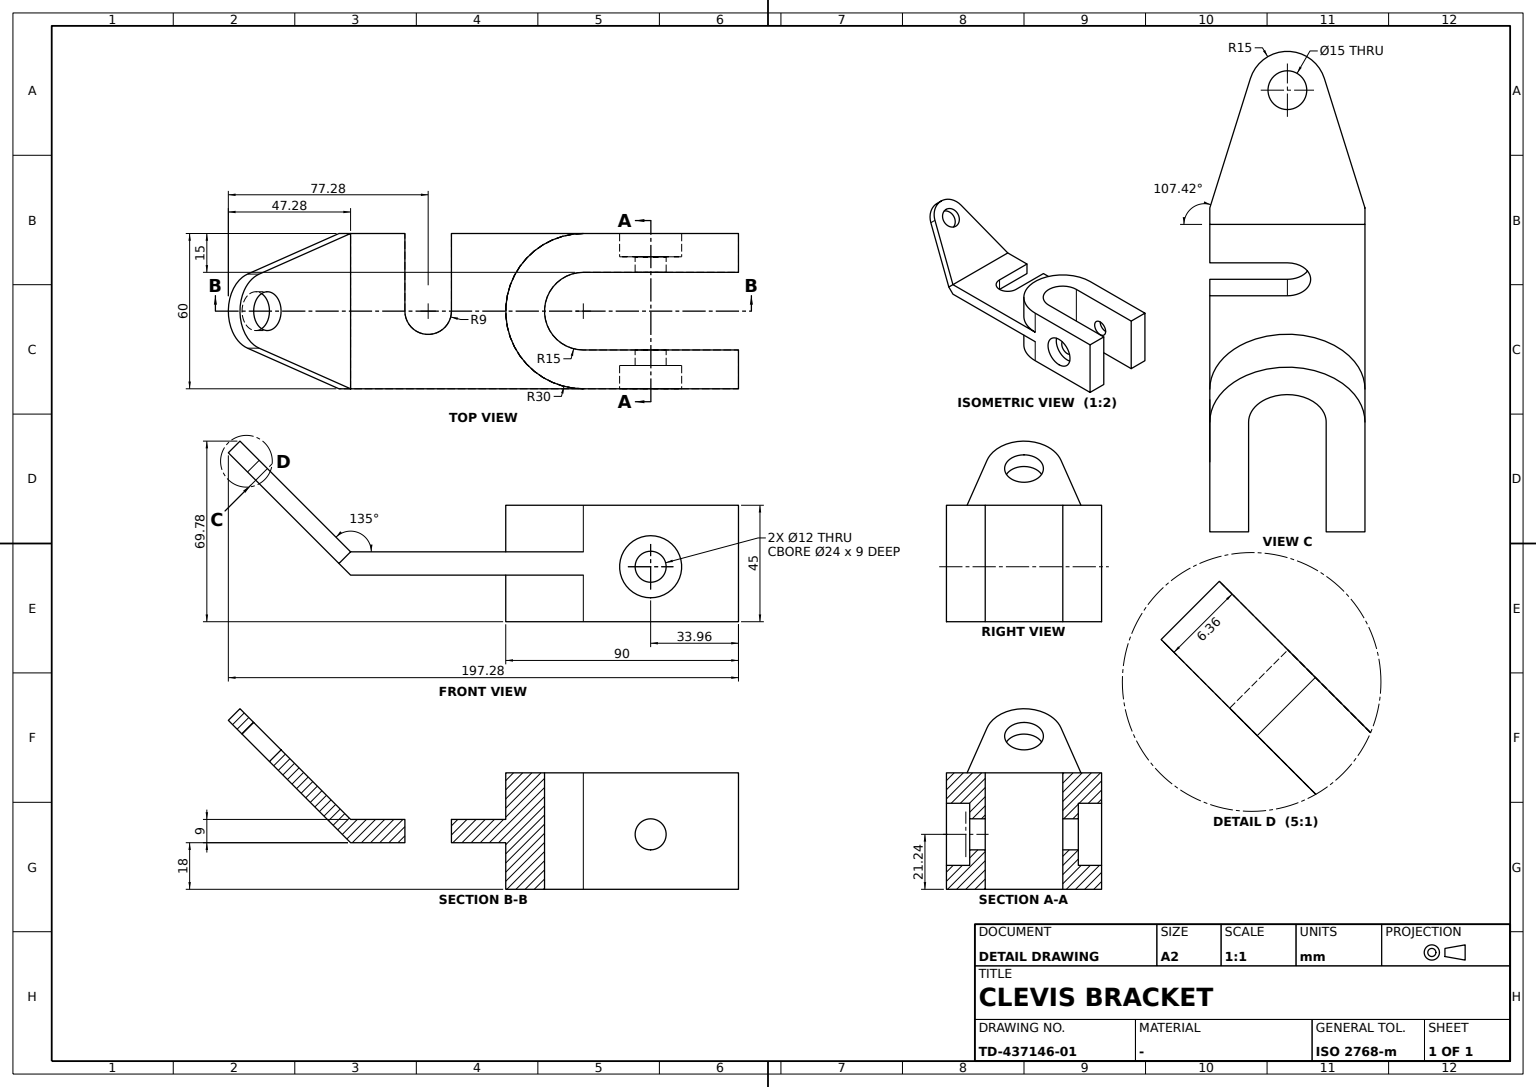
ISO-10303-21;
HEADER;
FILE_DESCRIPTION((''),'2;1');
FILE_NAME('','',(''),(''),'','','');
FILE_SCHEMA(('AUTOMOTIVE_DESIGN'));
ENDSEC;
DATA;
#1=APPLICATION_CONTEXT('');
#2=PRODUCT_CONTEXT('',#1,'mechanical');
#3=PRODUCT('','','',(#2));
#4=PRODUCT_DEFINITION_FORMATION('','',#3);
#5=PRODUCT_DEFINITION_CONTEXT('',#1,'design');
#6=PRODUCT_DEFINITION('','',#4,#5);
#7=PRODUCT_DEFINITION_SHAPE('','',#6);
#8=(LENGTH_UNIT()NAMED_UNIT(*)SI_UNIT(.MILLI.,.METRE.));
#9=(NAMED_UNIT(*)PLANE_ANGLE_UNIT()SI_UNIT($,.RADIAN.));
#10=(NAMED_UNIT(*)SI_UNIT($,.STERADIAN.)SOLID_ANGLE_UNIT());
#11=UNCERTAINTY_MEASURE_WITH_UNIT(LENGTH_MEASURE(0.005),#8,'distance_accuracy_value','');
#12=(GEOMETRIC_REPRESENTATION_CONTEXT(3)GLOBAL_UNCERTAINTY_ASSIGNED_CONTEXT((#11))GLOBAL_UNIT_ASSIGNED_CONTEXT((#8,#9,#10))REPRESENTATION_CONTEXT('',''));
#13=CARTESIAN_POINT('',(-30.,0.,4.5));
#14=VERTEX_POINT('',#13);
#15=CARTESIAN_POINT('',(-30.,-51.,4.5));
#16=VERTEX_POINT('',#15);
#17=DIRECTION('',(0.,-1.,0.));
#18=VECTOR('',#17,1000.);
#19=LINE('',#13,#18);
#20=EDGE_CURVE('',#14,#16,#19,.T.);
#21=ORIENTED_EDGE('',*,*,#20,.T.);
#22=CARTESIAN_POINT('',(0.,-51.,4.5));
#23=VERTEX_POINT('',#22);
#24=DIRECTION('',(-1.,0.,0.));
#25=VECTOR('',#24,1000.);
#26=LINE('',#22,#25);
#27=EDGE_CURVE('',#23,#16,#26,.T.);
#28=ORIENTED_EDGE('',*,*,#27,.F.);
#29=CARTESIAN_POINT('',(0.,-69.,4.5));
#30=VERTEX_POINT('',#29);
#31=CARTESIAN_POINT('',(0.,-60.,4.5));
#32=DIRECTION('',(0.,0.,1.));
#33=DIRECTION('',(1.,0.,0.));
#34=AXIS2_PLACEMENT_3D('',#31,#32,#33);
#35=CIRCLE('',#34,9.);
#36=EDGE_CURVE('',#30,#23,#35,.T.);
#37=ORIENTED_EDGE('',*,*,#36,.F.);
#38=CARTESIAN_POINT('',(-30.,-69.,4.5));
#39=VERTEX_POINT('',#38);
#40=VECTOR('',#33,1000.);
#41=LINE('',#38,#40);
#42=EDGE_CURVE('',#39,#30,#41,.T.);
#43=ORIENTED_EDGE('',*,*,#42,.F.);
#44=CARTESIAN_POINT('',(-30.,-90.,4.5));
#45=VERTEX_POINT('',#44);
#46=EDGE_CURVE('',#39,#45,#19,.T.);
#47=ORIENTED_EDGE('',*,*,#46,.T.);
#48=CARTESIAN_POINT('',(30.,-90.,4.5));
#49=VERTEX_POINT('',#48);
#50=CARTESIAN_POINT('',(0.,-90.,4.5));
#51=LINE('',#50,#25);
#52=EDGE_CURVE('',#49,#45,#51,.T.);
#53=ORIENTED_EDGE('',*,*,#52,.F.);
#54=CARTESIAN_POINT('',(30.,0.,4.5));
#55=VERTEX_POINT('',#54);
#56=LINE('',#54,#18);
#57=EDGE_CURVE('',#55,#49,#56,.T.);
#58=ORIENTED_EDGE('',*,*,#57,.F.);
#59=CARTESIAN_POINT('',(0.,0.,4.5));
#60=AXIS2_PLACEMENT_3D('',#59,#32,#33);
#61=CIRCLE('',#60,30.);
#62=EDGE_CURVE('',#14,#55,#61,.T.);
#63=ORIENTED_EDGE('',*,*,#62,.F.);
#64=EDGE_LOOP('',(#21,#28,#37,#43,#47,#53,#58,#63));
#65=FACE_BOUND('',#64,.T.);
#66=DIRECTION('',(0.,1.,0.));
#67=AXIS2_PLACEMENT_3D('',#59,#32,#66);
#68=PLANE('',#67);
#69=ADVANCED_FACE('',(#65),#68,.T.);
#70=ORIENTED_EDGE('',*,*,#36,.T.);
#71=CARTESIAN_POINT('',(0.,-51.,-4.5));
#72=VERTEX_POINT('',#71);
#73=CARTESIAN_POINT('',(0.,-51.,-9.66));
#74=VECTOR('',#32,1000.);
#75=LINE('',#73,#74);
#76=EDGE_CURVE('',#23,#72,#75,.F.);
#77=ORIENTED_EDGE('',*,*,#76,.T.);
#78=CARTESIAN_POINT('',(0.,-69.,-4.5));
#79=VERTEX_POINT('',#78);
#80=CARTESIAN_POINT('',(0.,-60.,-4.5));
#81=AXIS2_PLACEMENT_3D('',#80,#32,#33);
#82=CIRCLE('',#81,9.);
#83=EDGE_CURVE('',#79,#72,#82,.T.);
#84=ORIENTED_EDGE('',*,*,#83,.F.);
#85=CARTESIAN_POINT('',(0.,-69.,-9.66));
#86=LINE('',#85,#74);
#87=EDGE_CURVE('',#30,#79,#86,.F.);
#88=ORIENTED_EDGE('',*,*,#87,.F.);
#89=EDGE_LOOP('',(#70,#77,#84,#88));
#90=FACE_BOUND('',#89,.T.);
#91=CARTESIAN_POINT('',(0.,-60.,-9.66));
#92=AXIS2_PLACEMENT_3D('',#91,#32,#66);
#93=CYLINDRICAL_SURFACE('',#92,9.);
#94=ADVANCED_FACE('',(#90),#93,.F.);
#95=CARTESIAN_POINT('',(-30.,0.,22.5));
#96=VERTEX_POINT('',#95);
#97=CARTESIAN_POINT('',(30.,0.,22.5));
#98=VERTEX_POINT('',#97);
#99=CARTESIAN_POINT('',(0.,0.,22.5));
#100=AXIS2_PLACEMENT_3D('',#99,#32,#33);
#101=CIRCLE('',#100,30.);
#102=EDGE_CURVE('',#96,#98,#101,.T.);
#103=ORIENTED_EDGE('',*,*,#102,.F.);
#104=CARTESIAN_POINT('',(-30.,0.,0.));
#105=LINE('',#104,#74);
#106=EDGE_CURVE('',#14,#96,#105,.T.);
#107=ORIENTED_EDGE('',*,*,#106,.F.);
#108=ORIENTED_EDGE('',*,*,#62,.T.);
#109=CARTESIAN_POINT('',(30.,0.,0.));
#110=LINE('',#109,#74);
#111=EDGE_CURVE('',#55,#98,#110,.T.);
#112=ORIENTED_EDGE('',*,*,#111,.T.);
#113=EDGE_LOOP('',(#103,#107,#108,#112));
#114=FACE_BOUND('',#113,.T.);
#115=CARTESIAN_POINT('',(0.,0.,0.));
#116=AXIS2_PLACEMENT_3D('',#115,#32,#66);
#117=CYLINDRICAL_SURFACE('',#116,30.);
#118=ADVANCED_FACE('',(#114),#117,.T.);
#119=CARTESIAN_POINT('',(21.,26.036339,10.741734));
#120=VERTEX_POINT('',#119);
#121=CARTESIAN_POINT('',(21.,26.036339,-1.258266));
#122=AXIS2_PLACEMENT_3D('',#121,#24,#32);
#123=CIRCLE('',#122,12.);
#124=EDGE_CURVE('',#120,#120,#123,.T.);
#125=ORIENTED_EDGE('',*,*,#124,.F.);
#126=EDGE_LOOP('',(#125));
#127=FACE_BOUND('',#126,.T.);
#128=CARTESIAN_POINT('',(21.,26.036339,4.741734));
#129=VERTEX_POINT('',#128);
#130=CIRCLE('',#122,6.);
#131=EDGE_CURVE('',#129,#129,#130,.T.);
#132=ORIENTED_EDGE('',*,*,#131,.T.);
#133=EDGE_LOOP('',(#132));
#134=FACE_BOUND('',#133,.T.);
#135=CARTESIAN_POINT('',(21.,32.036339,-1.258266));
#136=AXIS2_PLACEMENT_3D('',#135,#24,#66);
#137=PLANE('',#136);
#138=ADVANCED_FACE('',(#127,#134),#137,.F.);
#139=ORIENTED_EDGE('',*,*,#124,.T.);
#140=EDGE_LOOP('',(#139));
#141=FACE_BOUND('',#140,.T.);
#142=CARTESIAN_POINT('',(30.,26.036339,-13.258266));
#143=VERTEX_POINT('',#142);
#144=CARTESIAN_POINT('',(30.,26.036339,-1.258266));
#145=DIRECTION('',(0.,0.,-1.));
#146=AXIS2_PLACEMENT_3D('',#144,#33,#145);
#147=CIRCLE('',#146,12.);
#148=EDGE_CURVE('',#143,#143,#147,.T.);
#149=ORIENTED_EDGE('',*,*,#148,.T.);
#150=EDGE_LOOP('',(#149));
#151=FACE_BOUND('',#150,.T.);
#152=CARTESIAN_POINT('',(-29.9,26.036339,-1.258266));
#153=AXIS2_PLACEMENT_3D('',#152,#33,#66);
#154=CYLINDRICAL_SURFACE('',#153,12.);
#155=ADVANCED_FACE('',(#141,#151),#154,.F.);
#156=CARTESIAN_POINT('',(-15.,60.,22.5));
#157=VERTEX_POINT('',#156);
#158=CARTESIAN_POINT('',(-15.,0.,22.5));
#159=VERTEX_POINT('',#158);
#160=LINE('',#156,#18);
#161=EDGE_CURVE('',#157,#159,#160,.T.);
#162=ORIENTED_EDGE('',*,*,#161,.F.);
#163=CARTESIAN_POINT('',(-30.,60.,22.5));
#164=VERTEX_POINT('',#163);
#165=CARTESIAN_POINT('',(0.,60.,22.5));
#166=LINE('',#165,#40);
#167=EDGE_CURVE('',#164,#157,#166,.T.);
#168=ORIENTED_EDGE('',*,*,#167,.F.);
#169=LINE('',#95,#18);
#170=EDGE_CURVE('',#164,#96,#169,.T.);
#171=ORIENTED_EDGE('',*,*,#170,.T.);
#172=ORIENTED_EDGE('',*,*,#102,.T.);
#173=CARTESIAN_POINT('',(30.,60.,22.5));
#174=VERTEX_POINT('',#173);
#175=VECTOR('',#66,1000.);
#176=LINE('',#97,#175);
#177=EDGE_CURVE('',#98,#174,#176,.T.);
#178=ORIENTED_EDGE('',*,*,#177,.T.);
#179=CARTESIAN_POINT('',(15.,60.,22.5));
#180=VERTEX_POINT('',#179);
#181=EDGE_CURVE('',#180,#174,#166,.T.);
#182=ORIENTED_EDGE('',*,*,#181,.F.);
#183=CARTESIAN_POINT('',(15.,0.,22.5));
#184=VERTEX_POINT('',#183);
#185=LINE('',#183,#175);
#186=EDGE_CURVE('',#184,#180,#185,.T.);
#187=ORIENTED_EDGE('',*,*,#186,.F.);
#188=CIRCLE('',#100,15.);
#189=EDGE_CURVE('',#159,#184,#188,.T.);
#190=ORIENTED_EDGE('',*,*,#189,.F.);
#191=EDGE_LOOP('',(#162,#168,#171,#172,#178,#182,#187,#190));
#192=FACE_BOUND('',#191,.T.);
#193=AXIS2_PLACEMENT_3D('',#99,#32,#66);
#194=PLANE('',#193);
#195=ADVANCED_FACE('',(#192),#194,.T.);
#196=CARTESIAN_POINT('',(14.311818,-125.349193,39.849193));
#197=VERTEX_POINT('',#196);
#198=CARTESIAN_POINT('',(14.311818,-129.849193,35.349193));
#199=VERTEX_POINT('',#198);
#200=CARTESIAN_POINT('',(14.311818,-243.121687,-77.9233));
#201=DIRECTION('',(0.,0.707106781,0.707106781));
#202=VECTOR('',#201,1000.);
#203=LINE('',#200,#202);
#204=EDGE_CURVE('',#197,#199,#203,.F.);
#205=ORIENTED_EDGE('',*,*,#204,.T.);
#206=CARTESIAN_POINT('',(30.,-94.5,0.));
#207=VERTEX_POINT('',#206);
#208=CARTESIAN_POINT('',(31.818079,-90.403437,-4.096563));
#209=DIRECTION('',(-0.299420588,-0.674665588,0.674665588));
#210=VECTOR('',#209,1000.);
#211=LINE('',#208,#210);
#212=EDGE_CURVE('',#207,#199,#211,.T.);
#213=ORIENTED_EDGE('',*,*,#212,.F.);
#214=CARTESIAN_POINT('',(30.,-47.25,47.25));
#215=DIRECTION('',(0.,-0.707106781,-0.707106781));
#216=VECTOR('',#215,1000.);
#217=LINE('',#214,#216);
#218=EDGE_CURVE('',#49,#207,#217,.T.);
#219=ORIENTED_EDGE('',*,*,#218,.F.);
#220=LINE('',#48,#210);
#221=EDGE_CURVE('',#49,#197,#220,.T.);
#222=ORIENTED_EDGE('',*,*,#221,.T.);
#223=EDGE_LOOP('',(#205,#213,#219,#222));
#224=FACE_BOUND('',#223,.T.);
#225=DIRECTION('',(0.954121225,-0.211722328,0.211722328));
#226=AXIS2_PLACEMENT_3D('',#48,#225,#209);
#227=PLANE('',#226);
#228=ADVANCED_FACE('',(#224),#227,.T.);
#229=CARTESIAN_POINT('',(-14.311818,-125.349193,39.849193));
#230=VERTEX_POINT('',#229);
#231=CARTESIAN_POINT('',(-14.311818,-129.849193,35.349193));
#232=VERTEX_POINT('',#231);
#233=CARTESIAN_POINT('',(-14.311818,-243.121687,-77.9233));
#234=LINE('',#233,#202);
#235=EDGE_CURVE('',#230,#232,#234,.F.);
#236=ORIENTED_EDGE('',*,*,#235,.T.);
#237=CARTESIAN_POINT('',(0.,-126.673359,32.173359));
#238=DIRECTION('',(0.,0.707106781,-0.707106781));
#239=AXIS2_PLACEMENT_3D('',#237,#215,#238);
#240=CIRCLE('',#239,15.);
#241=EDGE_CURVE('',#199,#232,#240,.T.);
#242=ORIENTED_EDGE('',*,*,#241,.F.);
#243=ORIENTED_EDGE('',*,*,#204,.F.);
#244=CARTESIAN_POINT('',(0.,-122.173359,36.673359));
#245=DIRECTION('',(0.,-0.707106781,0.707106781));
#246=AXIS2_PLACEMENT_3D('',#244,#201,#245);
#247=CIRCLE('',#246,15.);
#248=EDGE_CURVE('',#230,#197,#247,.T.);
#249=ORIENTED_EDGE('',*,*,#248,.F.);
#250=EDGE_LOOP('',(#236,#242,#243,#249));
#251=FACE_BOUND('',#250,.T.);
#252=CARTESIAN_POINT('',(0.,-239.945852,-81.099135));
#253=AXIS2_PLACEMENT_3D('',#252,#201,#24);
#254=CYLINDRICAL_SURFACE('',#253,15.);
#255=ADVANCED_FACE('',(#251),#254,.T.);
#256=CARTESIAN_POINT('',(-30.,0.,-22.5));
#257=VERTEX_POINT('',#256);
#258=CARTESIAN_POINT('',(30.,0.,-22.5));
#259=VERTEX_POINT('',#258);
#260=CARTESIAN_POINT('',(0.,0.,-22.5));
#261=AXIS2_PLACEMENT_3D('',#260,#32,#33);
#262=CIRCLE('',#261,30.);
#263=EDGE_CURVE('',#257,#259,#262,.T.);
#264=ORIENTED_EDGE('',*,*,#263,.T.);
#265=CARTESIAN_POINT('',(30.,0.,-4.5));
#266=VERTEX_POINT('',#265);
#267=EDGE_CURVE('',#259,#266,#110,.T.);
#268=ORIENTED_EDGE('',*,*,#267,.T.);
#269=CARTESIAN_POINT('',(-30.,0.,-4.5));
#270=VERTEX_POINT('',#269);
#271=CARTESIAN_POINT('',(0.,0.,-4.5));
#272=AXIS2_PLACEMENT_3D('',#271,#32,#33);
#273=CIRCLE('',#272,30.);
#274=EDGE_CURVE('',#270,#266,#273,.T.);
#275=ORIENTED_EDGE('',*,*,#274,.F.);
#276=EDGE_CURVE('',#257,#270,#105,.T.);
#277=ORIENTED_EDGE('',*,*,#276,.F.);
#278=EDGE_LOOP('',(#264,#268,#275,#277));
#279=FACE_BOUND('',#278,.T.);
#280=ADVANCED_FACE('',(#279),#117,.T.);
#281=CARTESIAN_POINT('',(-30.,-69.,-4.5));
#282=VERTEX_POINT('',#281);
#283=CARTESIAN_POINT('',(-30.,-90.,-4.5));
#284=VERTEX_POINT('',#283);
#285=LINE('',#269,#18);
#286=EDGE_CURVE('',#282,#284,#285,.T.);
#287=ORIENTED_EDGE('',*,*,#286,.T.);
#288=CARTESIAN_POINT('',(-30.,-94.5,0.));
#289=VERTEX_POINT('',#288);
#290=CARTESIAN_POINT('',(-30.,-17.25,-77.25));
#291=VECTOR('',#245,1000.);
#292=LINE('',#290,#291);
#293=EDGE_CURVE('',#284,#289,#292,.T.);
#294=ORIENTED_EDGE('',*,*,#293,.T.);
#295=CARTESIAN_POINT('',(-30.,-17.25,77.25));
#296=LINE('',#295,#216);
#297=EDGE_CURVE('',#45,#289,#296,.T.);
#298=ORIENTED_EDGE('',*,*,#297,.F.);
#299=ORIENTED_EDGE('',*,*,#46,.F.);
#300=CARTESIAN_POINT('',(-30.,-69.,0.));
#301=VECTOR('',#145,1000.);
#302=LINE('',#300,#301);
#303=EDGE_CURVE('',#39,#282,#302,.T.);
#304=ORIENTED_EDGE('',*,*,#303,.T.);
#305=EDGE_LOOP('',(#287,#294,#298,#299,#304));
#306=FACE_BOUND('',#305,.T.);
#307=CARTESIAN_POINT('',(-30.,60.,0.));
#308=AXIS2_PLACEMENT_3D('',#307,#24,#17);
#309=PLANE('',#308);
#310=ADVANCED_FACE('',(#306),#309,.T.);
#311=CARTESIAN_POINT('',(0.,-121.370058,26.870058));
#312=VERTEX_POINT('',#311);
#313=CIRCLE('',#239,7.5);
#314=EDGE_CURVE('',#312,#312,#313,.T.);
#315=ORIENTED_EDGE('',*,*,#314,.T.);
#316=EDGE_LOOP('',(#315));
#317=FACE_BOUND('',#316,.T.);
#318=CARTESIAN_POINT('',(0.,-127.476659,41.976659));
#319=VERTEX_POINT('',#318);
#320=CIRCLE('',#246,7.5);
#321=EDGE_CURVE('',#319,#319,#320,.T.);
#322=ORIENTED_EDGE('',*,*,#321,.T.);
#323=EDGE_LOOP('',(#322));
#324=FACE_BOUND('',#323,.T.);
#325=CARTESIAN_POINT('',(0.,-146.560203,12.286514));
#326=AXIS2_PLACEMENT_3D('',#325,#201,#24);
#327=CYLINDRICAL_SURFACE('',#326,7.5);
#328=ADVANCED_FACE('',(#317,#324),#327,.F.);
#329=ORIENTED_EDGE('',*,*,#218,.T.);
#330=CARTESIAN_POINT('',(30.,-90.,-4.5));
#331=VERTEX_POINT('',#330);
#332=LINE('',#330,#291);
#333=EDGE_CURVE('',#331,#207,#332,.T.);
#334=ORIENTED_EDGE('',*,*,#333,.F.);
#335=LINE('',#265,#18);
#336=EDGE_CURVE('',#266,#331,#335,.T.);
#337=ORIENTED_EDGE('',*,*,#336,.F.);
#338=ORIENTED_EDGE('',*,*,#267,.F.);
#339=CARTESIAN_POINT('',(30.,60.,-22.5));
#340=VERTEX_POINT('',#339);
#341=LINE('',#258,#175);
#342=EDGE_CURVE('',#259,#340,#341,.T.);
#343=ORIENTED_EDGE('',*,*,#342,.T.);
#344=CARTESIAN_POINT('',(30.,60.,0.));
#345=LINE('',#344,#74);
#346=EDGE_CURVE('',#340,#174,#345,.T.);
#347=ORIENTED_EDGE('',*,*,#346,.T.);
#348=ORIENTED_EDGE('',*,*,#177,.F.);
#349=ORIENTED_EDGE('',*,*,#111,.F.);
#350=ORIENTED_EDGE('',*,*,#57,.T.);
#351=EDGE_LOOP('',(#329,#334,#337,#338,#343,#347,#348,#349,#350));
#352=FACE_BOUND('',#351,.T.);
#353=ORIENTED_EDGE('',*,*,#148,.F.);
#354=EDGE_LOOP('',(#353));
#355=FACE_BOUND('',#354,.T.);
#356=AXIS2_PLACEMENT_3D('',#109,#33,#66);
#357=PLANE('',#356);
#358=ADVANCED_FACE('',(#352,#355),#357,.T.);
#359=CARTESIAN_POINT('',(15.,60.,-22.5));
#360=VERTEX_POINT('',#359);
#361=CARTESIAN_POINT('',(0.,60.,-22.5));
#362=LINE('',#361,#40);
#363=EDGE_CURVE('',#360,#340,#362,.T.);
#364=ORIENTED_EDGE('',*,*,#363,.F.);
#365=CARTESIAN_POINT('',(15.,60.,0.));
#366=LINE('',#365,#301);
#367=EDGE_CURVE('',#180,#360,#366,.T.);
#368=ORIENTED_EDGE('',*,*,#367,.F.);
#369=ORIENTED_EDGE('',*,*,#181,.T.);
#370=ORIENTED_EDGE('',*,*,#346,.F.);
#371=EDGE_LOOP('',(#364,#368,#369,#370));
#372=FACE_BOUND('',#371,.T.);
#373=AXIS2_PLACEMENT_3D('',#307,#17,#33);
#374=PLANE('',#373);
#375=ADVANCED_FACE('',(#372),#374,.F.);
#376=ORIENTED_EDGE('',*,*,#42,.T.);
#377=ORIENTED_EDGE('',*,*,#87,.T.);
#378=LINE('',#281,#40);
#379=EDGE_CURVE('',#282,#79,#378,.T.);
#380=ORIENTED_EDGE('',*,*,#379,.F.);
#381=ORIENTED_EDGE('',*,*,#303,.F.);
#382=EDGE_LOOP('',(#376,#377,#380,#381));
#383=FACE_BOUND('',#382,.T.);
#384=AXIS2_PLACEMENT_3D('',#38,#66,#33);
#385=PLANE('',#384);
#386=ADVANCED_FACE('',(#383),#385,.T.);
#387=ORIENTED_EDGE('',*,*,#235,.F.);
#388=DIRECTION('',(0.299420588,-0.674665588,0.674665588));
#389=VECTOR('',#388,1000.);
#390=LINE('',#44,#389);
#391=EDGE_CURVE('',#45,#230,#390,.T.);
#392=ORIENTED_EDGE('',*,*,#391,.F.);
#393=ORIENTED_EDGE('',*,*,#297,.T.);
#394=CARTESIAN_POINT('',(-26.438918,-102.523963,8.023963));
#395=LINE('',#394,#389);
#396=EDGE_CURVE('',#289,#232,#395,.T.);
#397=ORIENTED_EDGE('',*,*,#396,.T.);
#398=EDGE_LOOP('',(#387,#392,#393,#397));
#399=FACE_BOUND('',#398,.T.);
#400=DIRECTION('',(0.954121225,0.211722328,-0.211722328));
#401=AXIS2_PLACEMENT_3D('',#44,#400,#388);
#402=PLANE('',#401);
#403=ADVANCED_FACE('',(#399),#402,.F.);
#404=ORIENTED_EDGE('',*,*,#76,.F.);
#405=ORIENTED_EDGE('',*,*,#27,.T.);
#406=CARTESIAN_POINT('',(-30.,-51.,-4.5));
#407=VERTEX_POINT('',#406);
#408=LINE('',#15,#301);
#409=EDGE_CURVE('',#16,#407,#408,.T.);
#410=ORIENTED_EDGE('',*,*,#409,.T.);
#411=LINE('',#71,#40);
#412=EDGE_CURVE('',#407,#72,#411,.T.);
#413=ORIENTED_EDGE('',*,*,#412,.T.);
#414=EDGE_LOOP('',(#404,#405,#410,#413));
#415=FACE_BOUND('',#414,.T.);
#416=AXIS2_PLACEMENT_3D('',#22,#17,#24);
#417=PLANE('',#416);
#418=ADVANCED_FACE('',(#415),#417,.T.);
#419=CARTESIAN_POINT('',(-30.,26.036339,10.741734));
#420=VERTEX_POINT('',#419);
#421=CARTESIAN_POINT('',(-30.,26.036339,-1.258266));
#422=AXIS2_PLACEMENT_3D('',#421,#24,#32);
#423=CIRCLE('',#422,12.);
#424=EDGE_CURVE('',#420,#420,#423,.T.);
#425=ORIENTED_EDGE('',*,*,#424,.T.);
#426=EDGE_LOOP('',(#425));
#427=FACE_BOUND('',#426,.T.);
#428=CARTESIAN_POINT('',(-21.,26.036339,-13.258266));
#429=VERTEX_POINT('',#428);
#430=CARTESIAN_POINT('',(-21.,26.036339,-1.258266));
#431=AXIS2_PLACEMENT_3D('',#430,#33,#145);
#432=CIRCLE('',#431,12.);
#433=EDGE_CURVE('',#429,#429,#432,.T.);
#434=ORIENTED_EDGE('',*,*,#433,.T.);
#435=EDGE_LOOP('',(#434));
#436=FACE_BOUND('',#435,.T.);
#437=ADVANCED_FACE('',(#427,#436),#154,.F.);
#438=ORIENTED_EDGE('',*,*,#321,.F.);
#439=EDGE_LOOP('',(#438));
#440=FACE_BOUND('',#439,.T.);
#441=ORIENTED_EDGE('',*,*,#391,.T.);
#442=ORIENTED_EDGE('',*,*,#248,.T.);
#443=ORIENTED_EDGE('',*,*,#221,.F.);
#444=ORIENTED_EDGE('',*,*,#52,.T.);
#445=EDGE_LOOP('',(#441,#442,#443,#444));
#446=FACE_BOUND('',#445,.T.);
#447=CARTESIAN_POINT('',(30.,-132.77996,47.27996));
#448=AXIS2_PLACEMENT_3D('',#447,#201,#238);
#449=PLANE('',#448);
#450=ADVANCED_FACE('',(#440,#446),#449,.T.);
#451=CARTESIAN_POINT('',(-15.,26.036339,-7.258266));
#452=VERTEX_POINT('',#451);
#453=CARTESIAN_POINT('',(-15.,26.036339,-1.258266));
#454=AXIS2_PLACEMENT_3D('',#453,#33,#145);
#455=CIRCLE('',#454,6.);
#456=EDGE_CURVE('',#452,#452,#455,.T.);
#457=ORIENTED_EDGE('',*,*,#456,.T.);
#458=EDGE_LOOP('',(#457));
#459=FACE_BOUND('',#458,.T.);
#460=CARTESIAN_POINT('',(-21.,26.036339,-7.258266));
#461=VERTEX_POINT('',#460);
#462=CIRCLE('',#431,6.);
#463=EDGE_CURVE('',#461,#461,#462,.T.);
#464=ORIENTED_EDGE('',*,*,#463,.F.);
#465=EDGE_LOOP('',(#464));
#466=FACE_BOUND('',#465,.T.);
#467=CARTESIAN_POINT('',(29.9,26.036339,-1.258266));
#468=AXIS2_PLACEMENT_3D('',#467,#24,#66);
#469=CYLINDRICAL_SURFACE('',#468,6.);
#470=ADVANCED_FACE('',(#459,#466),#469,.F.);
#471=CARTESIAN_POINT('',(15.,26.036339,4.741734));
#472=VERTEX_POINT('',#471);
#473=CARTESIAN_POINT('',(15.,26.036339,-1.258266));
#474=AXIS2_PLACEMENT_3D('',#473,#24,#32);
#475=CIRCLE('',#474,6.);
#476=EDGE_CURVE('',#472,#472,#475,.T.);
#477=ORIENTED_EDGE('',*,*,#476,.T.);
#478=EDGE_LOOP('',(#477));
#479=FACE_BOUND('',#478,.T.);
#480=ORIENTED_EDGE('',*,*,#131,.F.);
#481=EDGE_LOOP('',(#480));
#482=FACE_BOUND('',#481,.T.);
#483=ADVANCED_FACE('',(#479,#482),#469,.F.);
#484=CARTESIAN_POINT('',(-15.,0.,-22.5));
#485=VERTEX_POINT('',#484);
#486=CARTESIAN_POINT('',(-15.,0.,-0.66));
#487=LINE('',#486,#74);
#488=EDGE_CURVE('',#159,#485,#487,.F.);
#489=ORIENTED_EDGE('',*,*,#488,.F.);
#490=ORIENTED_EDGE('',*,*,#189,.T.);
#491=CARTESIAN_POINT('',(15.,0.,-22.5));
#492=VERTEX_POINT('',#491);
#493=CARTESIAN_POINT('',(15.,0.,-0.66));
#494=LINE('',#493,#74);
#495=EDGE_CURVE('',#184,#492,#494,.F.);
#496=ORIENTED_EDGE('',*,*,#495,.T.);
#497=CIRCLE('',#261,15.);
#498=EDGE_CURVE('',#485,#492,#497,.T.);
#499=ORIENTED_EDGE('',*,*,#498,.F.);
#500=EDGE_LOOP('',(#489,#490,#496,#499));
#501=FACE_BOUND('',#500,.T.);
#502=CARTESIAN_POINT('',(0.,0.,-0.66));
#503=AXIS2_PLACEMENT_3D('',#502,#32,#66);
#504=CYLINDRICAL_SURFACE('',#503,15.);
#505=ADVANCED_FACE('',(#501),#504,.F.);
#506=CARTESIAN_POINT('',(-30.,60.,-22.5));
#507=VERTEX_POINT('',#506);
#508=CARTESIAN_POINT('',(-15.,60.,-22.5));
#509=VERTEX_POINT('',#508);
#510=EDGE_CURVE('',#507,#509,#362,.T.);
#511=ORIENTED_EDGE('',*,*,#510,.F.);
#512=LINE('',#307,#74);
#513=EDGE_CURVE('',#507,#164,#512,.T.);
#514=ORIENTED_EDGE('',*,*,#513,.T.);
#515=ORIENTED_EDGE('',*,*,#167,.T.);
#516=LINE('',#156,#301);
#517=EDGE_CURVE('',#157,#509,#516,.T.);
#518=ORIENTED_EDGE('',*,*,#517,.T.);
#519=EDGE_LOOP('',(#511,#514,#515,#518));
#520=FACE_BOUND('',#519,.T.);
#521=ADVANCED_FACE('',(#520),#374,.F.);
#522=ORIENTED_EDGE('',*,*,#498,.T.);
#523=LINE('',#491,#18);
#524=EDGE_CURVE('',#360,#492,#523,.T.);
#525=ORIENTED_EDGE('',*,*,#524,.F.);
#526=ORIENTED_EDGE('',*,*,#363,.T.);
#527=ORIENTED_EDGE('',*,*,#342,.F.);
#528=ORIENTED_EDGE('',*,*,#263,.F.);
#529=LINE('',#256,#18);
#530=EDGE_CURVE('',#507,#257,#529,.T.);
#531=ORIENTED_EDGE('',*,*,#530,.F.);
#532=ORIENTED_EDGE('',*,*,#510,.T.);
#533=LINE('',#508,#18);
#534=EDGE_CURVE('',#509,#485,#533,.T.);
#535=ORIENTED_EDGE('',*,*,#534,.T.);
#536=EDGE_LOOP('',(#522,#525,#526,#527,#528,#531,#532,#535));
#537=FACE_BOUND('',#536,.T.);
#538=AXIS2_PLACEMENT_3D('',#260,#32,#66);
#539=PLANE('',#538);
#540=ADVANCED_FACE('',(#537),#539,.F.);
#541=LINE('',#330,#25);
#542=EDGE_CURVE('',#331,#284,#541,.T.);
#543=ORIENTED_EDGE('',*,*,#542,.F.);
#544=ORIENTED_EDGE('',*,*,#333,.T.);
#545=ORIENTED_EDGE('',*,*,#212,.T.);
#546=ORIENTED_EDGE('',*,*,#241,.T.);
#547=ORIENTED_EDGE('',*,*,#396,.F.);
#548=ORIENTED_EDGE('',*,*,#293,.F.);
#549=EDGE_LOOP('',(#543,#544,#545,#546,#547,#548));
#550=FACE_BOUND('',#549,.T.);
#551=ORIENTED_EDGE('',*,*,#314,.F.);
#552=EDGE_LOOP('',(#551));
#553=FACE_BOUND('',#552,.T.);
#554=AXIS2_PLACEMENT_3D('',#330,#215,#245);
#555=PLANE('',#554);
#556=ADVANCED_FACE('',(#550,#553),#555,.T.);
#557=ORIENTED_EDGE('',*,*,#513,.F.);
#558=ORIENTED_EDGE('',*,*,#530,.T.);
#559=ORIENTED_EDGE('',*,*,#276,.T.);
#560=EDGE_CURVE('',#270,#407,#285,.T.);
#561=ORIENTED_EDGE('',*,*,#560,.T.);
#562=ORIENTED_EDGE('',*,*,#409,.F.);
#563=ORIENTED_EDGE('',*,*,#20,.F.);
#564=ORIENTED_EDGE('',*,*,#106,.T.);
#565=ORIENTED_EDGE('',*,*,#170,.F.);
#566=EDGE_LOOP('',(#557,#558,#559,#561,#562,#563,#564,#565));
#567=FACE_BOUND('',#566,.T.);
#568=ORIENTED_EDGE('',*,*,#424,.F.);
#569=EDGE_LOOP('',(#568));
#570=FACE_BOUND('',#569,.T.);
#571=ADVANCED_FACE('',(#567,#570),#309,.T.);
#572=ORIENTED_EDGE('',*,*,#534,.F.);
#573=ORIENTED_EDGE('',*,*,#517,.F.);
#574=ORIENTED_EDGE('',*,*,#161,.T.);
#575=ORIENTED_EDGE('',*,*,#488,.T.);
#576=EDGE_LOOP('',(#572,#573,#574,#575));
#577=FACE_BOUND('',#576,.T.);
#578=ORIENTED_EDGE('',*,*,#456,.F.);
#579=EDGE_LOOP('',(#578));
#580=FACE_BOUND('',#579,.T.);
#581=AXIS2_PLACEMENT_3D('',#156,#33,#17);
#582=PLANE('',#581);
#583=ADVANCED_FACE('',(#577,#580),#582,.T.);
#584=ORIENTED_EDGE('',*,*,#433,.F.);
#585=EDGE_LOOP('',(#584));
#586=FACE_BOUND('',#585,.T.);
#587=ORIENTED_EDGE('',*,*,#463,.T.);
#588=EDGE_LOOP('',(#587));
#589=FACE_BOUND('',#588,.T.);
#590=CARTESIAN_POINT('',(-21.,32.036339,-1.258266));
#591=AXIS2_PLACEMENT_3D('',#590,#33,#66);
#592=PLANE('',#591);
#593=ADVANCED_FACE('',(#586,#589),#592,.F.);
#594=ORIENTED_EDGE('',*,*,#495,.F.);
#595=ORIENTED_EDGE('',*,*,#186,.T.);
#596=ORIENTED_EDGE('',*,*,#367,.T.);
#597=ORIENTED_EDGE('',*,*,#524,.T.);
#598=EDGE_LOOP('',(#594,#595,#596,#597));
#599=FACE_BOUND('',#598,.T.);
#600=ORIENTED_EDGE('',*,*,#476,.F.);
#601=EDGE_LOOP('',(#600));
#602=FACE_BOUND('',#601,.T.);
#603=AXIS2_PLACEMENT_3D('',#183,#24,#66);
#604=PLANE('',#603);
#605=ADVANCED_FACE('',(#599,#602),#604,.T.);
#606=ORIENTED_EDGE('',*,*,#286,.F.);
#607=ORIENTED_EDGE('',*,*,#379,.T.);
#608=ORIENTED_EDGE('',*,*,#83,.T.);
#609=ORIENTED_EDGE('',*,*,#412,.F.);
#610=ORIENTED_EDGE('',*,*,#560,.F.);
#611=ORIENTED_EDGE('',*,*,#274,.T.);
#612=ORIENTED_EDGE('',*,*,#336,.T.);
#613=ORIENTED_EDGE('',*,*,#542,.T.);
#614=EDGE_LOOP('',(#606,#607,#608,#609,#610,#611,#612,#613));
#615=FACE_BOUND('',#614,.T.);
#616=AXIS2_PLACEMENT_3D('',#271,#32,#66);
#617=PLANE('',#616);
#618=ADVANCED_FACE('',(#615),#617,.F.);
#619=CLOSED_SHELL('',(#69,#94,#118,#138,#155,#195,#228,#255,#280,#310,#328,#358,#375,#386,#403,#418,#437,#450,#470,#483,#505,#521,#540,#556,#571,#583,#593,#605,#618));
#620=MANIFOLD_SOLID_BREP('',#619);
#621=ADVANCED_BREP_SHAPE_REPRESENTATION('',(#620),#12);
#622=SHAPE_DEFINITION_REPRESENTATION(#7,#621);
ENDSEC;
END-ISO-10303-21;
